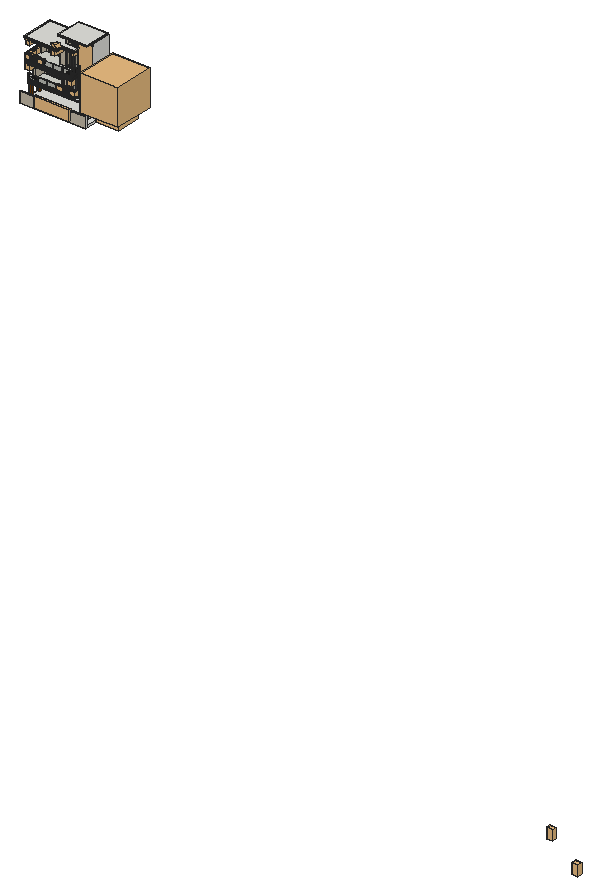
# SketchUp Ruby script. Lengths in inches.
U = 1.inch
M = Sketchup.active_model
def pt(a) = Geom::Point3d.new(a.map { |v| v * U })
def face(e, loops, mat)
  f = e.add_face(loops[0].map { |a| pt(a) })
  loops[1..].each { |l| e.add_face(l.map { |a| pt(a) }).erase! }
  f.material = f.back_material = mat if mat
  f
end
# faces: each face lists its corners as indices into pts; further lists are holes
def faces(e, pts, list, mat = nil) = list.each { |f| face(e, (f[0].is_a?(Array) ? f : [f]).map { |l| l.map { |i| pts[i] } }, mat) }
# xy, xz, yz: faces in a plane at the given z, y or x. An outline is a flat list of corners, or four numbers for a rectangle; further outlines are holes
def ring(l) = l.size == 4 ? [[l[0], l[1]], [l[2], l[1]], [l[2], l[3]], [l[0], l[3]]] : l.each_slice(2).to_a
def flat(e, list, mat, &to3) = list.each { |f| face(e, (f[0].is_a?(Array) ? f : [f]).map { |l| ring(l).map { |u, v| to3.(u, v) } }, mat) }
def xy(e, z, list, mat = nil) = flat(e, list, mat) { |x, y| [x, y, z] }
def xz(e, y, list, mat = nil) = flat(e, list, mat) { |x, z| [x, y, z] }
def yz(e, x, list, mat = nil) = flat(e, list, mat) { |y, z| [x, y, z] }
def lines(e, pts, list) = list.each { |a, b| e.add_line(pt(pts[a]), pt(pts[b])) }
# prism: a flat outline (further loops are holes) pulled along v
def prism(e, loops, v, mat = nil)
  f = face(e, loops, mat); d = Geom::Vector3d.new(v.map { |x| x * U })
  f.pushpull(f.normal.samedirection?(d) ? d.length : -d.length)
end
def box(e, o, s, mat = nil) = prism(e, [[o, [o[0] + s[0], o[1], o[2]], [o[0] + s[0], o[1] + s[1], o[2]], [o[0], o[1] + s[1], o[2]]]], [0, 0, s[2]], mat)
def at(x, y, z, deg = 0) = Geom::Transformation.translation(pt([x, y, z])) * Geom::Transformation.rotation(ORIGIN, Z_AXIS, deg.degrees)
def axes(o, x, y, z) = Geom::Transformation.new([*x, 0, *y, 0, *z, 0, *pt(o).to_a, 1])
def part(name) = M.definitions.add(name)
# library, detail: a bought-in or finely detailed component or shape, given as its bounding box
def library(name, o, s) = part(name).tap { |d| box(d.entities, o, s) }
def detail(e, o, s) = box(e.add_group.entities, o, s)
def put(e, d, t, mat = nil) = e.add_instance(d, t).tap { |i| i.material = mat if mat }
def group(e, t, mat = nil) = e.add_group.tap { |g| g.transformation = t; g.material = mat if mat }.entities
root = M.entities
M.materials.add("AM113_062_Tilia").color = [58, 81, 37]
M.materials.add("AM113_062_Tilia_Bark").color = [88, 85, 72]
M.materials.add("Aluminum_Anodized_DarkGray").color = [87, 83, 78]
M.materials.add("Aluminum_Polished").color = [83, 85, 85]
M.materials.add("Glass_Coated_Black").color = [65, 65, 65]
M.materials["Glass_Coated_Black"].alpha = 0.42
M.materials.add("Glass_Window_Neutral").color = [0, 0, 0]
M.materials["Glass_Window_Neutral"].alpha = 0.125
M.materials.add("Heather_Band").color = [45, 45, 45]
M.materials.add("Lily_Blonde").color = [255, 240, 201]
M.materials.add("Material__1").color = [190, 136, 85]
M.materials.add("Material__2").color = [51, 42, 44]
M.materials.add("Material__3").color = [119, 136, 107]
M.materials.add("Tiles White 02 160cm").color = [214, 215, 207]
M.materials.add("Windows").color = [58, 58, 58]
M.materials.add("Wood Planks Pecan 33-81 150cm").color = [83, 63, 40]
M.materials.add("[Color C08]").color = [102, 51, 0]
M.materials.add("[Color K01]").color = [194, 185, 166]
M.materials.add("[Color M06]").color = [86, 86, 86]
M.materials.add("[Color_000]").color = [255, 255, 255]
M.materials.add("[Metal Corrugated Shiny]1").color = [192, 192, 192]
c1 = part("Group\#54")
box(c1.entities,[0,0,0],[2,1,28])
c2 = part("Group\#56")
p = [[0.11,0.32,0.14],[0.11,0.69,0.14]]
lines(c2.entities,p,[[0,1]])
g1 = group(c2.entities,at(0.11,0,0))
prism(g1,[[[0,0.24,0],[0,0.32,0.14],[0,0.24,0.27],[0,0.08,0.27],[0,0,0.14],[0,0.08,0]]],[-0.11,0,0])
c3 = part("Ver Glass Railing")
g2 = group(c3.entities,at(0,0,0),"Aluminum_Polished")
box(g2,[0,0,0],[2,185,2])
g3 = group(c3.entities,at(0,0,2),"Aluminum_Polished")
p = [[1.41,1,0],[1.41,36.8,0],[1.41,184,0],[1.29,184,0],[1.29,1,0],[1.29,36.8,0],
  [1.41,184,28],[1.29,184,28],[1.41,148.2,28],[1.29,148.2,28],[1.41,1,28],[1.29,1,28],
  [1.29,111.4,28],[1.29,111.4,0],[1.41,111.4,0],[1.41,111.4,28],[1.29,110.4,0],[1.29,110.4,28],
  [1.41,110.4,28],[1.41,110.4,0],[1.29,74.6,28],[1.29,74.6,0],[1.41,74.6,0],[1.41,74.6,28],
  [1.29,73.6,0],[1.29,73.6,28],[1.41,73.6,28],[1.41,73.6,0],[1.29,148.2,0],[1.41,148.2,0],
  [1.29,147.2,0],[1.29,147.2,28],[1.41,147.2,28],[1.41,147.2,0],[1.29,37.8,28],[1.29,37.8,0],
  [1.41,37.8,0],[1.41,37.8,28],[1.29,36.8,28],[1.41,36.8,28]]
lines(g3,p,[[0,1],[2,3],[4,5],[6,7],[6,8],[7,9],[10,11],[2,6],[3,7],[0,4],[11,4],[10,0],
  [12,13],[14,15],[16,17],[18,19],[20,21],[22,23],[24,25],[26,27],[27,22],[24,21],[23,26],[20,25],
  [9,28],[29,8],[30,31],[32,33],[33,29],[30,28],[8,32],[9,31],[34,35],[36,37],[5,38],[39,1],
  [1,36],[5,35],[37,39],[14,33],[19,14],[22,19],[36,27],[13,30],[16,13],[21,16],[35,24],[15,18],
  [12,17],[29,2],[28,3],[18,23],[32,15],[17,20],[31,12],[26,37],[25,34],[34,38],[39,10],[38,11]])
g4 = group(g3,at(1.79,1,0))
box(g4,[-0.5,0,0],[0.125,183,28],"Glass_Window_Neutral")
g5 = group(g3,at(0,184,28))
box(g5,[0,-184,0],[2.5,185,1])
put(g3,c1,axes([2,185,28],[-1,0,0],[0,-1,0],[0,0,-1]))
put(g3,c1,axes([2,1,28],[-1,0,0],[0,-1,0],[0,0,-1]))
put(g3,c1,axes([2,111.4,28],[-1,0,0],[0,-1,0],[0,0,-1]))
put(g3,c1,axes([2,74.6,28],[-1,0,0],[0,-1,0],[0,0,-1]))
g6 = group(g3,at(2,148.2,28))
box(g6,[-2,-1,-28],[2,1,28])
put(g3,c1,axes([2,37.8,28],[-1,0,0],[0,-1,0],[0,0,-1]))
put(g3,c2,at(1.17,146.31,24.26))
put(g3,c2,axes([1.17,148.89,24.54],[1,0,0],[0,-1,0],[0,0,-1]))
put(g3,c2,axes([1.17,148.89,4.79],[1,0,0],[0,-1,0],[0,0,-1]))
put(g3,c2,at(1.17,146.31,4.51))
put(g3,c2,at(1.17,109.51,4.51))
put(g3,c2,axes([1.17,112.09,4.79],[1,0,0],[0,-1,0],[0,0,-1]))
put(g3,c2,axes([1.17,112.09,24.54],[1,0,0],[0,-1,0],[0,0,-1]))
put(g3,c2,at(1.17,109.51,24.26))
put(g3,c2,axes([1.17,75.29,24.54],[1,0,0],[0,-1,0],[0,0,-1]))
put(g3,c2,at(1.17,72.71,4.51))
put(g3,c2,axes([1.17,75.29,4.79],[1,0,0],[0,-1,0],[0,0,-1]))
put(g3,c2,at(1.17,72.71,24.26))
put(g3,c2,axes([1.17,38.49,24.54],[1,0,0],[0,-1,0],[0,0,-1]))
put(g3,c2,at(1.17,35.91,4.51))
put(g3,c2,axes([1.17,38.49,4.79],[1,0,0],[0,-1,0],[0,0,-1]))
put(g3,c2,at(1.17,35.91,24.26))
c4 = part("Group\#59")
xy(c4.entities,0,[[0,0,54,3]],"Aluminum_Anodized_DarkGray")
xy(c4.entities,2,[[2.25,0,51.75,1],[2.25,2,51.75,3]],"Aluminum_Anodized_DarkGray")
xy(c4.entities,3,[[3.375,1,14.625,1.5],[15.75,1,26.4375,1.5],[27.5625,1,38.25,1.5],[39.375,1,50.625,1.5],[3.375,1.5,14.625,2],
  [15.75,1.5,26.4375,2],[27.5625,1.5,38.25,2],[39.375,1.5,50.625,2]],"Aluminum_Anodized_DarkGray")
xy(c4.entities,99,[[3.375,1,14.625,1.5],[15.75,1,26.4375,1.5],[26.4375,1,27.5625,2],[27.5625,1,38.25,1.5],[38.25,1,39.375,2],
  [39.375,1,50.625,1.5],[3.375,1.5,14.625,2],[15.75,1.5,26.4375,2],[27.5625,1.5,38.25,2],[39.375,1.5,50.625,2]],"Aluminum_Anodized_DarkGray")
xy(c4.entities,100,[[2.25,0,51.75,1],[2.25,2,51.75,3]],"Aluminum_Anodized_DarkGray")
xy(c4.entities,102,[[0,0,54,3]],"Aluminum_Anodized_DarkGray")
xz(c4.entities,0,[[[0,0,54,102],[2.25,2,51.75,100]]],"Aluminum_Anodized_DarkGray")
xz(c4.entities,1,[[[2.25,2,51.75,100],[3.375,3,14.625,99],[39.375,3,50.625,99],[27.5625,3,38.25,99],[15.75,3,26.4375,99]]],"Aluminum_Anodized_DarkGray")
xz(c4.entities,1.5,[[3.375,3,14.625,99],[15.75,3,27,99],[27.5625,3,38.8125,99],[39.375,3,50.625,99]],"Glass_Coated_Black")
xz(c4.entities,2,[[[2.25,2,51.75,100],[3.375,3,14.625,99],[39.375,3,50.625,99],[27.5625,3,38.25,99],[15.75,3,26.4375,99]]],"Aluminum_Anodized_DarkGray")
xz(c4.entities,3,[[[0,0,54,102],[2.25,2,51.75,100]]],"Aluminum_Anodized_DarkGray")
yz(c4.entities,0,[[0,0,3,102]],"Aluminum_Anodized_DarkGray")
yz(c4.entities,2.25,[[0,2,1,100],[2,2,3,100]],"Aluminum_Anodized_DarkGray")
yz(c4.entities,3.375,[[1,3,1.5,99],[1.5,3,2,99]],"Aluminum_Anodized_DarkGray")
yz(c4.entities,14.625,[[1,3,1.5,99],[1.5,3,2,99]],"Aluminum_Anodized_DarkGray")
yz(c4.entities,15.75,[[1,3,1.5,99],[1.5,3,2,99]],"Aluminum_Anodized_DarkGray")
yz(c4.entities,26.4375,[[1,3,2,99]],"Aluminum_Anodized_DarkGray")
yz(c4.entities,27.5625,[[1,3,1.5,99],[1.5,3,2,99]],"Aluminum_Anodized_DarkGray")
yz(c4.entities,38.25,[[1,3,2,99]],"Aluminum_Anodized_DarkGray")
yz(c4.entities,39.375,[[1,3,1.5,99],[1.5,3,2,99]],"Aluminum_Anodized_DarkGray")
yz(c4.entities,50.625,[[1,3,1.5,99],[1.5,3,2,99]],"Aluminum_Anodized_DarkGray")
yz(c4.entities,51.75,[[0,2,1,100],[2,2,3,100]],"Aluminum_Anodized_DarkGray")
yz(c4.entities,54,[[0,0,3,102]],"Aluminum_Anodized_DarkGray")
p = [[15.75,2,99],[14.625,2,99]]
lines(c4.entities,p,[[0,1]])
c5 = part("Untitled (2)")
put(c5.entities,c4,at(51.4375,0,0))
c6 = library("Back Drop",[0,0,0],[82.68,2.27,107.48])
c7 = part("Window+06")
g7 = group(c7.entities,at(-11,5.5,0,-90))
xy(g7,0,[[0,11,5.5,35]],"Windows")
xy(g7,2,[[0,13,5.5,33]],"Windows")
xy(g7,53,[[0,13,5.5,33]],"Windows")
xy(g7,55,[[0,11,5.5,35]],"Windows")
xz(g7,11,[[0,0,5.5,55]],"Windows")
xz(g7,13,[[0,2,5.5,53]],"Windows")
xz(g7,33,[[0,2,5.5,53]],"Windows")
xz(g7,35,[[0,0,5.5,55]],"Windows")
yz(g7,0,[[[11,0,35,55],[13,2,33,53]]],"Windows")
yz(g7,5.5,[[[11,0,35,55],[13,2,33,53]]],"Windows")
g8 = group(g7,at(2.75,2,2))
xy(g8,0,[[0,11,2,31]],"Windows")
xy(g8,1,[[0,12,1,30],[1,12,2,30]],"Windows")
xy(g8,25,[[0,12,1,30],[1,12,2,30]],"Windows")
xy(g8,26,[[0,11,2,31]],"Windows")
xz(g8,11,[[0,0,2,26]],"Windows")
xz(g8,12,[[0,1,1,25],[1,1,2,25]],"Windows")
xz(g8,30,[[0,1,1,25],[1,1,2,25]],"Windows")
xz(g8,31,[[0,0,2,26]],"Windows")
yz(g8,0,[[[11,0,31,26],[12,1,30,25]]],"Windows")
yz(g8,1,[[12,1,30,25]])
yz(g8,2,[[[11,0,31,26],[12,1,30,25]]],"Windows")
g9 = group(g7,at(0.75,2,27))
xy(g9,0,[[0,11,2,31]],"Windows")
xy(g9,1,[[0,12,1,30],[1,12,2,30]],"Windows")
xy(g9,25,[[0,12,1,30],[1,12,2,30]],"Windows")
xy(g9,26,[[0,11,2,31]],"Windows")
xz(g9,11,[[0,0,2,26]],"Windows")
xz(g9,12,[[0,1,1,25],[1,1,2,25]],"Windows")
xz(g9,30,[[0,1,1,25],[1,1,2,25]],"Windows")
xz(g9,31,[[0,0,2,26]],"Windows")
yz(g9,0,[[[11,0,31,26],[12,1,30,25]]],"Windows")
yz(g9,1,[[12,1,30,25]])
yz(g9,2,[[[11,0,31,26],[12,1,30,25]]],"Windows")
c8 = part("Untitled (2)\#1")
put(c8.entities,c4,at(51.4375,0,0))
c9 = library("Gate 243 022",[-149.15,-8.9,0],[298.3,17.8,91.39])
c10 = library("\#2",[-119.83,-119.83,113.8],[239.66,239.66,17.4])
c11 = library("\#4",[-204.92,-212.35,-236.71],[424.28,257.5,472.53])
c12 = part("\#3")
put(c12.entities,c11,axes([-0.37,309.72,0],[1.36765,0,0],[0,1.36765,0],[0,0,1.36765]),"Material__3")
c13 = library("\#1",[-174.07,-174.07,0],[348.14,348.14,140])
c14 = part("9")
put(c14.entities,c10,at(-19.94,-24.66,0),"Material__2")
put(c14.entities,c12,axes([17.67,-32.6,40.29],[0.29694,0.9549,0],[-0.21403,0.06656,0.97456],[0.9306,-0.28939,0.22414]))
put(c14.entities,c13,at(-19.94,-24.66,0),"Material__1")
c15 = part("Plant")
xy(c15.entities,0,[[6.51,0.48,5,0.62,3.57,1.15,2.33,2.03,1.36,3.2,0.73,4.58,0.48,6.08,0.62,7.59,1.15,9.02,2.03,10.26,3.2,11.23,4.58,11.86,6.08,12.11,7.59,11.97,9.02,11.4375,10.26,10.56,11.23,9.39,11.86,8.01,12.11,6.51,11.97,5,11.4375,3.57,10.56,2.33,9.39,1.36,8.01,0.73]],"[Metal Corrugated Shiny]1")
xy(c15.entities,0.86,[[[6.53,0,4.89,0.15,3.35,0.73,2.01,1.68,0.96,2.95,0.27,4.44,0,6.0625,0.15,7.7,0.73,9.24,1.68,10.58,2.95,11.63,4.44,12.32,6.0625,12.59,7.7,12.44,9.24,11.86,10.58,10.91,11.63,9.64,12.32,8.15,12.59,6.53,12.44,4.89,11.86,3.35,10.91,2.01,9.64,0.96,8.15,0.27],[6.51,0.48,8.01,0.73,9.39,1.36,10.56,2.33,11.4375,3.57,11.97,5,12.11,6.51,11.86,8.01,11.23,9.39,10.26,10.56,9.02,11.4375,7.59,11.97,6.08,12.11,4.58,11.86,3.2,11.23,2.03,10.26,1.15,9.02,0.62,7.59,0.48,6.08,0.73,4.58,1.36,3.2,2.33,2.03,3.57,1.15,5,0.62]]],"[Metal Corrugated Shiny]1")
xy(c15.entities,12.8125,[[6.5,0.69,7.94,0.9375,9.28,1.55,10.4,2.48,11.25,3.67,11.76,5.04,11.9,6.5,11.65,7.94,11.04,9.28,10.11,10.4,8.92,11.25,7.55,11.76,6.09,11.9,4.65,11.65,3.31,11.04,2.1875,10.11,1.34,8.92,0.83,7.55,0.69,6.09,0.9375,4.65,1.55,3.31,2.48,2.1875,3.67,1.34,5.04,0.83]])
xy(c15.entities,13.33,[[[6.52,0.3,8.06,0.56,9.48,1.21,10.69,2.21,11.6,3.49,12.15,4.96,12.29,6.52,12.03,8.06,11.38,9.48,10.38,10.69,9.1,11.6,7.63,12.15,6.07,12.29,4.53,12.03,3.11,11.38,1.9,10.38,0.99,9.1,0.44,7.63,0.3,6.07,0.56,4.53,1.21,3.11,2.21,1.9,3.49,0.99,4.96,0.44],[6.5,0.69,5.04,0.83,3.67,1.34,2.48,2.1875,1.55,3.31,0.9375,4.65,0.69,6.09,0.83,7.55,1.34,8.92,2.1875,10.11,3.31,11.04,4.65,11.65,6.09,11.9,7.55,11.76,8.92,11.25,10.11,10.4,11.04,9.28,11.65,7.94,11.9,6.5,11.76,5.04,11.25,3.67,10.4,2.48,9.28,1.55,7.94,0.9375]]],"[Color_000]")
xy(c15.entities,14.16,[[[6.53,0,8.15,0.27,9.64,0.96,10.91,2.01,11.86,3.35,12.44,4.89,12.59,6.53,12.32,8.15,11.63,9.64,10.58,10.91,9.24,11.86,7.7,12.44,6.0625,12.59,4.44,12.32,2.95,11.63,1.68,10.58,0.73,9.24,0.15,7.7,0,6.0625,0.27,4.44,0.96,2.95,2.01,1.68,3.35,0.73,4.89,0.15],[6.52,0.3,4.96,0.44,3.49,0.99,2.21,1.9,1.21,3.11,0.56,4.53,0.3,6.07,0.44,7.63,0.99,9.1,1.9,10.38,3.11,11.38,4.53,12.03,6.07,12.29,7.63,12.15,9.1,11.6,10.38,10.69,11.38,9.48,12.03,8.06,12.29,6.52,12.15,4.96,11.6,3.49,10.69,2.21,9.48,1.21,8.06,0.56]]],"[Metal Corrugated Shiny]1")
p = [[5,0.62,0],[6.51,0.48,0],[6.51,0.48,0.86],[5,0.62,0.86],[8.01,0.73,0],[8.01,0.73,0.86],
  [3.57,1.15,0],[3.57,1.15,0.86],[9.39,1.36,0],[9.39,1.36,0.86],[2.33,2.03,0],[2.33,2.03,0.86],
  [10.56,2.33,0],[10.56,2.33,0.86],[1.36,3.2,0],[1.36,3.2,0.86],[11.4375,3.57,0],[11.4375,3.57,0.86],
  [0.73,4.58,0],[0.73,4.58,0.86],[11.97,5,0],[11.97,5,0.86],[0.48,6.08,0],[0.48,6.08,0.86],
  [12.11,6.51,0],[12.11,6.51,0.86],[0.62,7.59,0],[0.62,7.59,0.86],[11.86,8.01,0],[11.86,8.01,0.86],
  [1.15,9.02,0],[1.15,9.02,0.86],[11.23,9.39,0],[11.23,9.39,0.86],[2.03,10.26,0],[2.03,10.26,0.86],
  [10.26,10.56,0],[10.26,10.56,0.86],[3.2,11.23,0],[3.2,11.23,0.86],[9.02,11.4375,0],[9.02,11.4375,0.86],
  [4.58,11.86,0],[4.58,11.86,0.86],[7.59,11.97,0],[7.59,11.97,0.86],[6.08,12.11,0],[6.08,12.11,0.86],
  [4.89,0.15,14.16],[4.89,0.15,0.86],[6.53,0,0.86],[6.53,0,14.16],[8.15,0.27,0.86],[8.15,0.27,14.16],
  [3.35,0.73,14.16],[3.35,0.73,0.86],[9.64,0.96,0.86],[9.64,0.96,14.16],[2.01,1.68,14.16],[2.01,1.68,0.86],
  [10.91,2.01,0.86],[10.91,2.01,14.16],[0.96,2.95,14.16],[0.96,2.95,0.86],[11.86,3.35,0.86],[11.86,3.35,14.16],
  [0.27,4.44,14.16],[0.27,4.44,0.86],[12.44,4.89,0.86],[12.44,4.89,14.16],[0,6.0625,14.16],[0,6.0625,0.86],
  [12.59,6.53,0.86],[12.59,6.53,14.16],[0.15,7.7,14.16],[0.15,7.7,0.86],[12.32,8.15,0.86],[12.32,8.15,14.16],
  [0.73,9.24,14.16],[0.73,9.24,0.86],[11.63,9.64,0.86],[11.63,9.64,14.16],[1.68,10.58,14.16],[1.68,10.58,0.86],
  [10.58,10.91,0.86],[10.58,10.91,14.16],[2.95,11.63,14.16],[2.95,11.63,0.86],[9.24,11.86,0.86],[9.24,11.86,14.16],
  [4.44,12.32,14.16],[4.44,12.32,0.86],[7.7,12.44,0.86],[7.7,12.44,14.16],[6.0625,12.59,14.16],[6.0625,12.59,0.86],
  [5.04,0.83,13.33],[6.5,0.69,13.33],[6.5,0.69,12.8125],[5.04,0.83,12.8125],[7.94,0.9375,13.33],[7.94,0.9375,12.8125],
  [3.67,1.34,13.33],[3.67,1.34,12.8125],[9.28,1.55,13.33],[9.28,1.55,12.8125],[2.48,2.1875,13.33],[2.48,2.1875,12.8125],
  [10.4,2.48,13.33],[10.4,2.48,12.8125],[1.55,3.31,13.33],[1.55,3.31,12.8125],[11.25,3.67,13.33],[11.25,3.67,12.8125],
  [0.9375,4.65,13.33],[0.9375,4.65,12.8125],[11.76,5.04,13.33],[11.76,5.04,12.8125],[0.69,6.09,13.33],[0.69,6.09,12.8125],
  [11.9,6.5,13.33],[11.9,6.5,12.8125],[0.83,7.55,13.33],[0.83,7.55,12.8125],[11.65,7.94,13.33],[11.65,7.94,12.8125],
  [1.34,8.92,13.33],[1.34,8.92,12.8125],[11.04,9.28,13.33],[11.04,9.28,12.8125],[2.1875,10.11,13.33],[2.1875,10.11,12.8125],
  [10.11,10.4,13.33],[10.11,10.4,12.8125],[3.31,11.04,13.33],[3.31,11.04,12.8125],[8.92,11.25,13.33],[8.92,11.25,12.8125],
  [4.65,11.65,13.33],[4.65,11.65,12.8125],[7.55,11.76,13.33],[7.55,11.76,12.8125],[6.09,11.9,13.33],[6.09,11.9,12.8125],
  [4.96,0.44,14.16],[6.52,0.3,14.16],[6.52,0.3,13.33],[4.96,0.44,13.33],[8.06,0.56,14.16],[8.06,0.56,13.33],
  [3.49,0.99,14.16],[3.49,0.99,13.33],[9.48,1.21,14.16],[9.48,1.21,13.33],[2.21,1.9,14.16],[2.21,1.9,13.33],
  [10.69,2.21,14.16],[10.69,2.21,13.33],[1.21,3.11,14.16],[1.21,3.11,13.33],[11.6,3.49,14.16],[11.6,3.49,13.33],
  [0.56,4.53,14.16],[0.56,4.53,13.33],[12.15,4.96,14.16],[12.15,4.96,13.33],[0.3,6.07,14.16],[0.3,6.07,13.33],
  [12.29,6.52,14.16],[12.29,6.52,13.33],[0.44,7.63,14.16],[0.44,7.63,13.33],[12.03,8.06,14.16],[12.03,8.06,13.33],
  [0.99,9.1,14.16],[0.99,9.1,13.33],[11.38,9.48,14.16],[11.38,9.48,13.33],[1.9,10.38,14.16],[1.9,10.38,13.33],
  [10.38,10.69,14.16],[10.38,10.69,13.33],[3.11,11.38,14.16],[3.11,11.38,13.33],[9.1,11.6,14.16],[9.1,11.6,13.33],
  [4.53,12.03,14.16],[4.53,12.03,13.33],[7.63,12.15,14.16],[7.63,12.15,13.33],[6.07,12.29,14.16],[6.07,12.29,13.33]]
faces(c15.entities,p,[[0,1,2,3],[1,4,5,2],[6,0,3,7],[4,8,9,5],[10,6,7,11],[8,12,13,9],[14,10,11,15],[12,16,17,13],
  [18,14,15,19],[16,20,21,17],[22,18,19,23],[20,24,25,21],[26,22,23,27],[24,28,29,25],[30,26,27,31],[28,32,33,29],
  [34,30,31,35],[32,36,37,33],[38,34,35,39],[36,40,41,37],[42,38,39,43],[40,44,45,41],[46,42,43,47],[44,46,47,45],
  [48,49,50,51],[51,50,52,53],[54,55,49,48],[53,52,56,57],[58,59,55,54],[57,56,60,61],[62,63,59,58],[61,60,64,65],
  [66,67,63,62],[65,64,68,69],[70,71,67,66],[69,68,72,73],[74,75,71,70],[73,72,76,77],[78,79,75,74],[77,76,80,81],
  [82,83,79,78],[81,80,84,85],[86,87,83,82],[85,84,88,89],[90,91,87,86],[89,88,92,93],[94,95,91,90],[93,92,95,94],
  [144,145,146,147],[145,148,149,146],[150,144,147,151],[148,152,153,149],[154,150,151,155],[152,156,157,153],[158,154,155,159],[156,160,161,157],
  [162,158,159,163],[160,164,165,161],[166,162,163,167],[164,168,169,165],[170,166,167,171],[168,172,173,169],[174,170,171,175],[172,176,177,173],
  [178,174,175,179],[176,180,181,177],[182,178,179,183],[180,184,185,181],[186,182,183,187],[184,188,189,185],[190,186,187,191],[188,190,191,189]],"[Metal Corrugated Shiny]1")
faces(c15.entities,p,[[96,97,98,99],[97,100,101,98],[102,96,99,103],[100,104,105,101],[106,102,103,107],[104,108,109,105],[110,106,107,111],[108,112,113,109],
  [114,110,111,115],[112,116,117,113],[118,114,115,119],[116,120,121,117],[122,118,119,123],[120,124,125,121],[126,122,123,127],[124,128,129,125],
  [130,126,127,131],[128,132,133,129],[134,130,131,135],[132,136,137,133],[138,134,135,139],[136,140,141,137],[142,138,139,143],[140,142,143,141]],"[Color_000]")
c16 = library("AM113_062_Tilia_Defintion",[-350.67,-364.73,-2.58],[672.29,726.36,1000])
c17 = library("AM113_062_Tilia_Defintion1",[-524.84,-500,219.37],[933.41,1000,877.77])
c18 = part("Group4\#1")
put(c18.entities,c16,axes([0,0,0],[0.28109,0,0],[0,0.28109,0],[0,0,0.28109]),"AM113_062_Tilia_Bark")
put(c18.entities,c17,axes([0,0,0],[0.33697,0,0],[0,0.33697,0],[0,0,0.33697]),"AM113_062_Tilia")
c19 = part("11")
put(c19.entities,c18,axes([919.91,680.74,314.96],[1,0,0],[0,0,-1],[0,1,0]))
c20 = library("Plante \#58",[-0.43,-1.58,0],[20.84,18.06,17.59])
c21 = library("climbing plant",[8874.76,-5589.78,-33.625],[50.13,38.07,87.16])
c22 = library("plant (1)",[-21.34,-27.21,-0.38],[41.91,41.15,38.97])
c23 = library("Group\#67",[0,0,0],[56.8,25.91,35.15])
xy(root,-17.125,[[0.11,0,548.05,13.1875]])
xy(root,-13.8125,[[115.18,0,410.1875,13.1875]])
xy(root,0,[[0.11,93.54,18.8,108.26],[475.9375,95.49,475.9375,265.11,18.8,265.11,18.8,268.74,0.11,268.74,0.11,305.14,500.93,305.14,500.93,95.49],[0.11,175.26,18.8,189.22],[0.11,249.72,18.8,268.74]])
xy(root,69.75,[[0.11,0,115.18,13.1875],[410.1875,0,548.05,13.1875]])
xy(root,97.5625,[[475.9375,81.24,500.93,95.49]])
xy(root,97.5625,[[0.11,81.24,0.11,93.54,18.8,93.54,18.8,108.26,0.11,108.26,0.11,175.26,18.8,175.26,18.8,189.22,0.11,189.22,0.11,249.72,18.8,249.72,18.8,265.11,475.9375,265.11,475.9375,81.24]],"Lily_Blonde")
xy(root,107.99,[[392.52,81.24,500.93,111.84]])
xy(root,118.375,[[392.52,111.84,451.25,148.65]])
xy(root,124.875,[[0.11,81.24,392.52,81.24,392.52,148.65,370.75,148.65,370.75,216.46,271.31,216.46,271.31,148.65,247.94,148.65,247.94,213.73,226.58,213.73,226.58,293.61,48.8,293.61,48.8,213.73,29.01,213.73,29.01,131.02,0.11,131.02]],"Tiles White 02 160cm")
xy(root,237.39,[[271.31,148.65,370.75,216.46]])
xy(root,240,[[48.8,213.73,226.58,293.61]],"Lily_Blonde")
xy(root,260.37,[[392.52,111.84,451.25,148.65]])
xy(root,260.37,[[0.11,45.35,0.11,131.02,29.01,131.02,29.01,213.73,247.94,213.73,247.94,148.65,392.52,148.65,392.52,45.35]],"Wood Planks Pecan 33-81 150cm")
xy(root,294.02,[[0.11,45.35,392.52,45.35,392.52,111.84,500.93,111.84,500.93,134.75,377.39,134.75,377.39,197.82,274.05,197.82,274.05,134.75,223.73,134.75,223.73,214.27,213.68,214.27,213.68,288.65,63.88,288.65,63.88,214.27,40.3,214.27,40.3,175.76,22.26,175.76,22.26,305.14,0.11,305.14]],"Tiles White 02 160cm")
xy(root,420.52,[[63.88,214.27,213.68,288.65]],"Lily_Blonde")
xy(root,444.72,[[274.05,134.75,377.39,197.82]],"Lily_Blonde")
xy(root,446.63,[[13.9,53.16,13.9,305.14,22.26,305.14,22.26,175.76,40.3,175.76,40.3,214.27,223.73,214.27,223.73,134.75,264.36,134.75,264.36,53.16]],"Wood Planks Pecan 33-81 150cm")
xy(root,446.63,[[5.625,40.51,5.625,305.14,13.9,305.14,13.9,53.16,264.36,53.16,264.36,134.75,377.39,134.75,377.39,88.86,272.74,88.86,272.74,40.51]],"[Color K01]")
xy(root,463.71,[[5.625,40.51,5.625,305.14,272.74,305.14,272.74,134.75,377.57,134.75,377.57,88.86,272.74,88.86,272.74,40.51]])
xy(root,463.71,[[0,34.88,0,305.14,5.625,305.14,5.625,40.51,272.74,40.51,272.74,88.86,377.57,88.86,377.57,134.75,383.19,134.75,383.19,83.23,278.36,83.23,278.36,34.88]],"[Color K01]")
xy(root,467.59,[[0,34.88,278.36,34.88,278.36,83.23,383.19,83.23,383.19,134.75,272.74,134.75,272.74,305.14,0,305.14]])
xy(root,483.54,[[295.32,134.75,377.39,166.63]])
xy(root,508.92,[[295.32,134.75,377.39,166.63]])
xy(root,531.31,[[272.74,134.75,488.2,305.14],[488.2,134.75,500.93,305.14]])
xy(root,531.31,[[242.875,90.67,242.875,305.14,272.74,305.14,272.74,134.75,488.2,134.75,488.2,90.67]],"Wood Planks Pecan 33-81 150cm")
xy(root,543.23,[[242.875,90.67,488.2,305.14]])
xz(root,0,[[0.11,-17.125,548.05,-17.125,548.05,69.75,410.1875,69.75,410.1875,-13.8125,115.18,-13.8125,115.18,69.75,0.11,69.75]],"[Color K01]")
xz(root,13.1875,[[0.11,-17.125,0.11,69.75,115.18,69.75,115.18,-13.8125,410.1875,-13.8125,410.1875,69.75,548.05,69.75,548.05,-17.125]])
xz(root,34.88,[[0,463.71,278.36,467.59]],"[Color K01]")
xz(root,40.51,[[5.625,446.63,272.74,463.71]],"Heather_Band")
xz(root,45.35,[[0.11,260.37,392.52,294.02]],"Heather_Band")
xz(root,81.24,[[0.11,97.5625,500.93,107.99],[0.11,107.99,392.52,118.375],[0.11,118.375,392.52,124.875]],"Heather_Band")
xz(root,83.23,[[278.36,463.71,383.19,467.59]],"[Color K01]")
xz(root,88.86,[[272.74,446.63,377.39,446.63,377.57,463.71,272.74,463.71]],"Heather_Band")
xz(root,90.67,[[242.875,531.31,488.2,543.23]],"Heather_Band")
xz(root,93.54,[[0.11,0,18.8,97.5625]],"[Color C08]")
xz(root,95.49,[[475.9375,0,500.93,97.5625]],"[Color C08]")
xz(root,108.26,[[0.11,0,18.8,97.5625]])
xz(root,111.84,[[392.52,107.99,500.93,107.99,500.93,116.43,451.25,116.43,451.25,118.375,392.52,118.375],[451.25,116.43,500.93,116.43,500.93,294.02,392.52,294.02,392.52,260.37,451.25,260.37]],"Heather_Band")
xz(root,131.02,[[0.11,124.875,29.01,260.37]],"[Color K01]")
xz(root,134.75,[[377.39,294.02,444.5625,294.02,444.5625,510.14,476.29,510.14,476.29,294.02,500.93,294.02,500.93,531.31,377.39,531.31,377.39,467.59,383.19,467.59,383.19,463.71,377.57,463.71,377.39,446.63],[444.5625,294.02,476.29,510.14],[377.39,446.63,377.57,463.71,377.39,463.71],[272.74,463.71,377.39,467.59],[377.39,463.71,383.19,467.59]])
xz(root,134.75,[[223.73,294.02,274.05,294.02,274.05,444.72,377.39,444.72,377.39,446.63,223.73,446.63],[272.74,467.59,377.39,467.59,377.39,483.54,295.32,483.54,295.32,508.92,377.39,508.92,377.39,531.31,272.74,531.31]],"[Color K01]")
xz(root,148.65,[[392.52,118.375,451.25,260.37]])
xz(root,148.65,[[247.94,124.875,271.31,124.875,271.31,237.39,370.75,237.39,370.75,124.875,392.52,124.875,392.52,260.37,247.94,260.37]],"[Color K01]")
xz(root,166.63,[[295.32,483.54,377.39,508.92]])
xz(root,175.26,[[0.11,0,18.8,97.5625]],"[Color C08]")
xz(root,175.76,[[22.26,294.02,40.3,446.63]],"[Color K01]")
xz(root,189.22,[[0.11,0,18.8,97.5625]])
xz(root,197.82,[[274.05,294.02,377.39,444.72]],"Lily_Blonde")
xz(root,213.73,[[29.01,124.875,48.8,124.875,48.8,240,226.58,240,226.58,124.875,247.94,124.875,247.94,260.37,29.01,260.37]],"[Color K01]")
xz(root,214.27,[[40.3,294.02,63.88,294.02,63.88,420.52,213.68,420.52,213.68,294.02,223.73,294.02,223.73,446.63,40.3,446.63]],"[Color K01]")
xz(root,216.46,[[271.31,124.875,370.75,237.39]])
xz(root,249.72,[[0.11,0,18.8,97.5625]],"[Color C08]")
xz(root,265.11,[[18.8,0,475.9375,97.5625]],"Lily_Blonde")
xz(root,268.74,[[0.11,0,18.8,97.5625]])
xz(root,288.65,[[63.88,294.02,213.68,420.52]],"Lily_Blonde")
xz(root,293.61,[[48.8,124.875,226.58,240]],"Lily_Blonde")
xz(root,305.14,[[0.11,0,0.11,294.02,22.26,294.02,22.26,446.63,500.93,446.63,500.93,0],[5.625,446.63,5.625,463.71,272.74,463.71,272.74,531.31,500.93,531.31,500.93,446.63],[0,463.71,272.74,467.59],[242.875,531.31,488.2,543.23]])
yz(root,0,[[34.88,463.71,305.14,467.59]])
yz(root,0.11,[[0,-17.125,13.1875,69.75],[93.54,0,108.26,97.5625],[175.26,0,189.22,97.5625],[249.72,0,268.74,97.5625],[268.74,0,305.14,97.5625],
  [81.24,97.5625,305.14,124.875],[131.02,124.875,131.02,260.37,45.35,260.37,45.35,294.02,305.14,294.02,305.14,124.875]])
yz(root,5.625,[[40.51,446.63,305.14,463.71]],"Heather_Band")
yz(root,18.8,[[265.11,0,268.74,97.5625]])
yz(root,18.8,[[93.54,0,108.26,97.5625],[175.26,0,189.22,97.5625],[249.72,0,265.11,97.5625]],"[Color C08]")
yz(root,22.26,[[175.76,294.02,305.14,446.63]])
yz(root,29.01,[[131.02,124.875,213.73,260.37]],"[Color K01]")
yz(root,40.3,[[175.76,294.02,214.27,446.63]],"[Color K01]")
yz(root,48.8,[[213.73,124.875,293.61,240]],"Lily_Blonde")
yz(root,63.88,[[214.27,294.02,288.65,420.52]],"Lily_Blonde")
yz(root,115.18,[[0,-13.8125,13.1875,69.75]])
yz(root,213.68,[[214.27,294.02,288.65,420.52]],"Lily_Blonde")
yz(root,223.73,[[134.75,294.02,214.27,446.63]],"[Color K01]")
yz(root,226.58,[[213.73,124.875,293.61,240]],"Lily_Blonde")
yz(root,242.875,[[90.67,531.31,305.14,543.23]])
yz(root,247.94,[[148.65,124.875,213.73,260.37]],"[Color K01]")
yz(root,271.31,[[148.65,124.875,216.46,237.39]])
yz(root,272.74,[[134.75,463.71,305.14,467.59],[134.75,467.59,305.14,531.31]])
yz(root,272.74,[[40.51,446.63,88.86,463.71]],"Heather_Band")
yz(root,274.05,[[134.75,294.02,197.82,444.72]],"Lily_Blonde")
yz(root,278.36,[[34.88,463.71,83.23,467.59]],"[Color K01]")
yz(root,295.32,[[134.75,483.54,166.63,508.92]])
yz(root,370.75,[[148.65,124.875,216.46,237.39]])
yz(root,377.39,[[134.75,483.54,166.63,508.92]])
yz(root,377.39,[[134.75,294.02,197.82,444.72]],"Lily_Blonde")
yz(root,383.19,[[83.23,463.71,134.75,467.59]],"[Color K01]")
yz(root,392.52,[[81.24,118.375,111.84,124.875],[111.84,118.375,148.65,124.875]])
yz(root,392.52,[[81.24,107.99,111.84,118.375],[45.35,260.37,111.84,272.48],[45.35,272.48,111.84,294.02]],"Heather_Band")
yz(root,410.1875,[[0,-13.8125,13.1875,69.75]])
yz(root,451.25,[[111.84,118.375,148.65,260.37]],"[Color K01]")
yz(root,475.9375,[[95.49,0,265.11,97.5625]])
yz(root,488.2,[[90.67,531.31,305.14,543.23]],"Heather_Band")
yz(root,500.93,[[95.49,0,305.14,0,305.14,116.43,111.84,116.43,111.84,107.99,81.24,107.99,81.24,97.5625,95.49,97.5625],[111.84,116.43,305.14,116.43,305.14,531.31,134.75,531.31,134.75,294.02,111.84,294.02]])
yz(root,548.05,[[0,-17.125,13.1875,69.75]])
p = [[377.39,88.86,446.63],[377.39,134.75,446.63],[377.57,134.75,463.71],[377.57,88.86,463.71]]
faces(root,p,[[0,1,2,3]],"Heather_Band")
put(root,c3,axes([0.11,45.35,294.02],[1,0,0],[0,1.40429,0],[0,0,1.5]))
put(root,c3,axes([392.52,45.35,294.02],[0,1,0],[-2.11031,0,0],[0,0,1.5]))
put(root,c3,axes([390.52,81.24,124.875],[0,1,0],[-2.11031,0,0],[0,0,1.5]))
put(root,c5,axes([-78.81,214.27,294.02],[2.77409,0,0],[0,1,0],[0,0,1.2402]))
put(root,c5,axes([-121.49,213.73,124.875],[3.30116,0,0],[0,1,0],[0,0,1.12868]))
put(root,c6,axes([377.79,132.48,294.02],[1.485,0,0],[0,1,0],[0,0,2.2]))
put(root,c7,axes([295.32,134.75,508.92],[0,0,-1.05729],[0,1,0],[1.52774,0,0]))
put(root,c8,axes([178.77,134.75,294.02],[1.88376,0,0],[0,1,0],[0,0,1.4774]))
put(root,c8,axes([176.59,148.65,124.875],[1.84144,0,0],[0,1,0],[0,0,1.10131]))
put(root,c3,axes([390.02,47.35,294.02],[1,0,0],[0,0.44987,0],[0,0,1.5]))
put(root,c6,axes([392.47,147.76,118.375],[0.70656,0,0],[0,0.39,0],[0,0,1.31333]))
put(root,c9,at(262.3,7.58,-13.85),"[Color M06]")
put(root,c14,axes([258.63,51.74,467.59],[0.0732,0,0],[0,0.0732,0],[0,0,0.0732]))
put(root,c15,at(359.33,58.09,295.35))
put(root,c15,at(31.86,112.89,123.88))
put(root,c19,axes([-240.84,483.45,-667.14],[1,0,0],[0,0,1],[0,-1,0]))
put(root,c15,at(12.62,112.69,123.88))
put(root,c15,at(343.89,58.09,295.35))
put(root,c20,axes([19.77,37.5,416.53],[1.572,0,0],[0,2.47148,0],[0,0,1.74]))
put(root,c20,axes([235.53,38.18,411.6875],[1.452,0,0],[0,4.6494,0],[0,0,2.0155]))
put(root,c20,axes([352.9,91.44,421.13],[1.2,0,0],[0,1.64,0],[0,0,1.45]))
put(root,c20,axes([357.38,47.93,225.43],[2.02176,0,0],[0,1.64,0],[0,0,1.9865]))
put(root,c20,axes([-0.85,51.37,215.93],[2.3352,0,0],[0,3.8212,0],[0,0,2.52633]))
put(root,c21,at(352.24,-175.43,7.45))
put(root,c22,at(233.28,195.82,124.875))
put(root,c21,at(0.11,0,69.75))
g10 = group(root,at(0.11,305.14,-17.125))
box(g10,[0,-291.96,0],[547.9375,291.96,17.125])
put(root,c23,at(2.11,45.35,297.9))
put(root,c23,at(47.77,45.35,297.02))
put(root,c23,at(91.93,45.94,297.02))
put(root,c23,at(335.83,81.24,127.875))
put(root,c23,at(235.2,81.24,128.75))
put(root,c23,at(287.39,81.24,128.75))
put(root,c23,at(5.66,213.17,297.9,-92.4))
put(root,c23,at(2.49,123.4,297.02,-92.4))
put(root,c23,at(3.75,167.55,297.02,-92.4))
